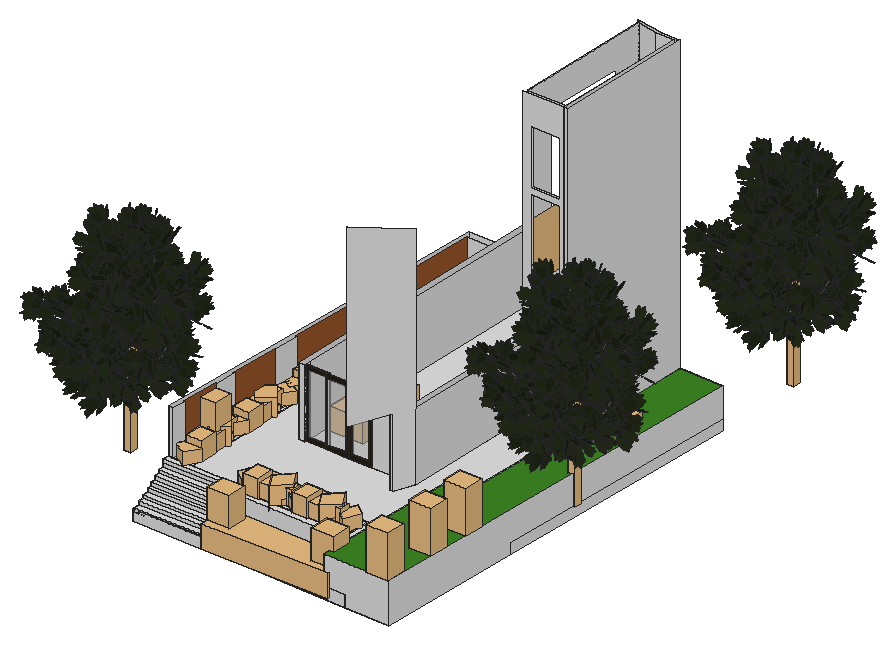
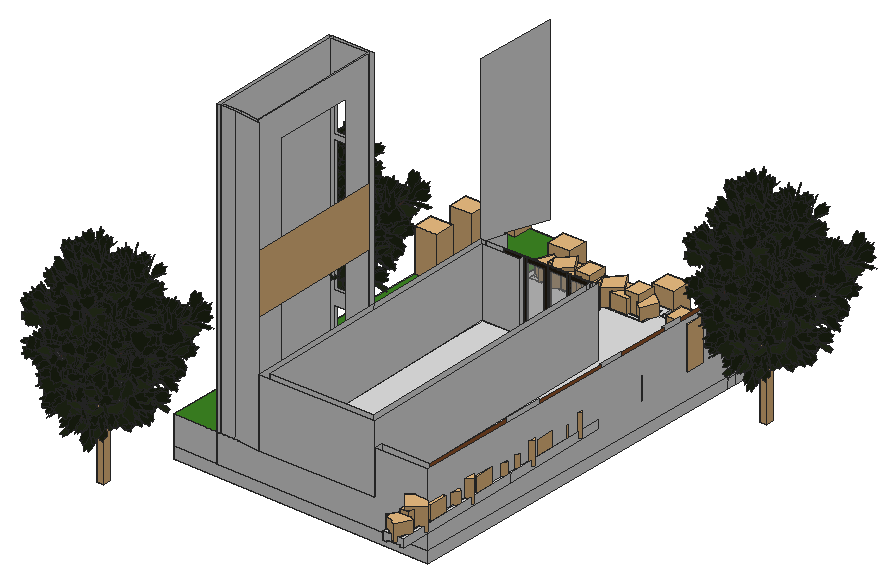
# SketchUp Ruby script. Lengths in inches.
U = 1.inch
M = Sketchup.active_model
def pt(a) = Geom::Point3d.new(a.map { |v| v * U })
def face(e, loops, mat)
  f = e.add_face(loops[0].map { |a| pt(a) })
  loops[1..].each { |l| e.add_face(l.map { |a| pt(a) }).erase! }
  f.material = f.back_material = mat if mat
  f
end
# faces: each face lists its corners as indices into pts; further lists are holes
def faces(e, pts, list, mat = nil) = list.each { |f| face(e, (f[0].is_a?(Array) ? f : [f]).map { |l| l.map { |i| pts[i] } }, mat) }
# xy, xz, yz: faces in a plane at the given z, y or x. An outline is a flat list of corners, or four numbers for a rectangle; further outlines are holes
def ring(l) = l.size == 4 ? [[l[0], l[1]], [l[2], l[1]], [l[2], l[3]], [l[0], l[3]]] : l.each_slice(2).to_a
def flat(e, list, mat, &to3) = list.each { |f| face(e, (f[0].is_a?(Array) ? f : [f]).map { |l| ring(l).map { |u, v| to3.(u, v) } }, mat) }
def xy(e, z, list, mat = nil) = flat(e, list, mat) { |x, y| [x, y, z] }
def xz(e, y, list, mat = nil) = flat(e, list, mat) { |x, z| [x, y, z] }
def yz(e, x, list, mat = nil) = flat(e, list, mat) { |y, z| [x, y, z] }
def lines(e, pts, list) = list.each { |a, b| e.add_line(pt(pts[a]), pt(pts[b])) }
# prism: a flat outline (further loops are holes) pulled along v
def prism(e, loops, v, mat = nil)
  f = face(e, loops, mat); d = Geom::Vector3d.new(v.map { |x| x * U })
  f.pushpull(f.normal.samedirection?(d) ? d.length : -d.length)
end
def box(e, o, s, mat = nil) = prism(e, [[o, [o[0] + s[0], o[1], o[2]], [o[0] + s[0], o[1] + s[1], o[2]], [o[0], o[1] + s[1], o[2]]]], [0, 0, s[2]], mat)
def at(x, y, z, deg = 0) = Geom::Transformation.translation(pt([x, y, z])) * Geom::Transformation.rotation(ORIGIN, Z_AXIS, deg.degrees)
def axes(o, x, y, z) = Geom::Transformation.new([*x, 0, *y, 0, *z, 0, *pt(o).to_a, 1])
def part(name) = M.definitions.add(name)
# library, detail: a bought-in or finely detailed component or shape, given as its bounding box
def library(name, o, s) = part(name).tap { |d| box(d.entities, o, s) }
def detail(e, o, s) = box(e.add_group.entities, o, s)
def put(e, d, t, mat = nil) = e.add_instance(d, t).tap { |i| i.material = mat if mat }
def group(e, t, mat = nil) = e.add_group.tap { |g| g.transformation = t; g.material = mat if mat }.entities
root = M.entities
M.materials.add("Green ash – green texture").color = [33, 41, 22]
M.materials.add("Material__1").color = [95, 70, 46]
M.materials.add("[Color A01]").color = [60, 133, 34]
M.materials.add("[Color M03]").color = [226, 226, 226]
M.materials.add("[Color_005]").color = [114, 114, 114]
M.materials.add("[Color_D09]").color = [86, 59, 49]
M.materials.add("[Translucent Glass Gray]2").color = [201, 201, 201]
M.materials["[Translucent Glass Gray]2"].alpha = 0.5
M.materials.add("[Wood Cherry Original]2").color = [152, 86, 42]
M.materials.add("oak swatch").color = [40, 31, 19]
c1 = part("Component\#13")
xz(c1.entities,0,[[2.54,0,9.87,0.64,10.99,2.07,11.4,3.42,15.13,2.28,14.48,4.31,16.14,5.21,16.14,6.08,19.81,7.28,19.6,9.67,17.45,11.49,17.45,12.16,18.82,14.37,17.48,14.37,14.41,13.66,14.41,15.23,12.5625,17.49,9.84,15.21,8.9,13.85,7.74,13.625,7.35,12.68,6.87,13.02,6.35,12.27,5.92,10.47,4.2,7.42,2.84,6.89,0,2.38,0.07,1.59,2.8125,4.94,3.37,3.59,2.54,3.37,2.12,2.22]],"Green ash – green texture")
c2 = part("Component\#14")
xz(c2.entities,0,[[1.1,0,1.61,0,2.73,1.11,4.34,2.72,5.21,6.36,5.85,7.16,6.35,6.9375,6.85,8.05,8.03,8.05,8.625,9.25,10.11,11.7,9.56,13.83,9.56,15.84,7.83,15.84,6.03,14.37,5.31,16.54,4.4375,17.39,1.45,14.31,0,9.15,1.4,5.18,3.01,6.08,1.98,1.39]],"Green ash – green texture")
c3 = part("Component\#16")
put(c3.entities,c1,axes([0,7.77,0],[1,0,0],[0,0.89571,0.44464],[0,-0.44464,0.89571]))
put(c3.entities,c2,axes([2.15,6.37,5.26],[0.57629,-0.80824,0.12095],[0.79263,0.51673,-0.3236],[0.19905,0.28236,0.93843]))
c4 = part("Component\#3")
put(c4.entities,c3,axes([-4.97,-3.22,4.05],[0.69883,-0.69034,0.18725],[0.53248,0.3273,-0.7806],[0.47759,0.64522,0.59632]))
c5 = part("Component\#4")
put(c5.entities,c4,axes([0,5.2,2.2],[1,0,0],[0,0.90259,0.43051],[0,-0.43051,0.90259]))
c6 = part("leaf group 2")
put(c6.entities,c5,axes([-11.99,4.41,-4.35],[2.22014,-0.82385,1.14017],[1.36501,1.77637,-1.37441],[-0.33979,1.75315,1.92841]))
c7 = part("Component\#5")
put(c7.entities,c6,axes([-5.27,11.65,1.68],[-0.48323,0.10636,-0.43072],[-0.11515,-0.64511,-0.03012],[-0.42845,0.05342,0.49388]))
c8 = part("Component\#15")
xz(c8.entities,0,[[0.64,0,0,0.1875,4.21,2.81,8.59,4.11,12.8,4.11,19.57,2.81,12.8,3.73,8.59,3.73,4.21,2.3125]],"[Color_D09]")
c9 = part("Leafy twig")
put(c9.entities,c7,axes([23.53,12.57,24.85],[0.06536,-0.90475,-0.42089],[0.61791,-0.2945,0.72901],[-0.78353,-0.30772,0.53981]))
put(c9.entities,c7,axes([22.7,12.25,24.83],[-0.47146,-0.89493,0.11311],[0.80135,-0.48549,-0.35888],[0.36776,-0.0521,0.90651]))
put(c9.entities,c7,axes([24.25,0.65,20.83],[0.8253,-0.50372,0.24924],[0.23848,0.71461,0.65749],[-0.51157,-0.48438,0.71194]))
put(c9.entities,c7,axes([23.54,-2.45,18.63],[0.04689,-0.92492,0.3511],[0.72122,-0.28285,-0.64421],[0.71641,0.2674,0.65188]))
put(c9.entities,c7,axes([22.39,16.15,27.04],[-0.5311,-0.82173,0.2419],[0.41574,0.01583,0.89559],[-0.77461,0.50499,0.40813]))
put(c9.entities,c8,axes([22.76,-5.09,13.48],[0,1.66539,0.44624],[-1.72414,0,0],[0,-0.44624,1.66539]))
c10 = part("Component\#12")
p = [[0,0,0.13],[0.41,0.77,0],[4.07,2.79,10.125],[3.73,2.15,10.23],[7.66,4.77,23.875],[7.4,4.27,23.96],
  [8.6875,5.26,35.99],[8.5,4.91,36.05],[8.32,4.9375,46.95],[8.21,4.74,46.98]]
faces(c10.entities,p,[[0,1,2,3],[3,2,4,5],[4,6,7,5],[6,8,9,7]],"[Color_005]")
c11 = part("Component\#2")
put(c11.entities,c10,axes([3.13,0.17,-0.45],[3.38032,6.88592,0.52481],[-5.85488,3.97559,0.303],[0,-1.35912,3.54524]))
put(c11.entities,c7,axes([0.37,31.375,148.94],[0.47772,0.64064,-1.51139],[2.85768,-0.62659,0.20284],[-0.43926,-3.3797,-0.3241]))
c12 = part("Tree branch")
put(c12.entities,c9,axes([28.11,72.66,46.26],[0.77413,-0.41274,-0.47998],[0.6311,0.56229,0.53435],[0.04934,-0.71657,0.69577]))
put(c12.entities,c9,axes([31.25,3.94,9.17],[0.73236,0.67893,0.05208],[-0.46223,0.55185,-0.69413],[-0.5,0.48428,0.71797]))
put(c12.entities,c9,axes([20.16,84.84,57.95],[0.96628,0.19619,0.16678],[-0.2575,0.73909,0.62245],[-0.00115,-0.6444,0.76469]))
put(c12.entities,c9,axes([30.13,29.18,11.93],[0.86603,0.2796,0.41452],[0,0.82904,-0.55919],[-0.5,0.48428,0.71797]))
put(c12.entities,c9,axes([47.67,28.63,-3.7],[0.1205,-0.71255,0.69119],[0.96646,0.24327,0.08231],[-0.2268,0.65809,0.71797]))
put(c12.entities,c9,axes([48.76,50.64,76.31],[-0.6716,0.46861,-0.57389],[0.01402,0.78248,0.62252],[0.74078,0.41004,-0.53209]))
put(c12.entities,c11,axes([42.34,0,10.34],[0.39368,0,0],[0,0.22544,-0.24092],[0,0.54032,0.50562]))
put(c12.entities,c9,axes([64.51,80.82,101.08],[-0.99604,0.06562,-0.06004],[-0.0106,0.58266,0.81265],[0.08831,0.81006,-0.57966]))
c13 = library("Component\#7",[-6.35,9.4375,-76.57],[12.56,13.68,315.77])
c14 = part("Component\#9")
put(c14.entities,c9,axes([-3.64,36.17,23.18],[0.95801,0.10249,0.26779],[-0.28581,0.41631,0.86313],[-0.02302,-0.90343,0.42812]))
put(c14.entities,c9,axes([13.16,55.79,39.92],[0.70711,-0.61725,0.34497],[0,0.48786,0.87292],[-0.70711,-0.61725,0.34497]))
put(c14.entities,c11,axes([18.8125,5.17,0.46],[0.25503,0,0],[0,0.20007,-0.0752],[0,0.16866,0.44872]))
put(c14.entities,c9,axes([23.62,-10.17,21.5],[-0.56253,0.81775,0.12181],[0.38738,0.13053,0.91263],[0.73041,0.56057,-0.39021]))
put(c14.entities,c9,axes([45.18,27.18,68.96],[-0.96593,-0.22593,0.12627],[0.12295,0.02876,0.992],[-0.22775,0.97372,0]))
c15 = part("Component\#10")
put(c15.entities,c11,axes([21.47,3.93,0.22],[0.25503,0,0],[0,0.21068,-0.03601],[0,0.08077,0.47252]))
put(c15.entities,c9,axes([-4.05,13.6875,55.34],[0.70711,0.70373,-0.069],[0,0.09758,0.99523],[0.70711,-0.70373,0.069]))
put(c15.entities,c9,axes([6.52,33.54,18.07],[0.92587,-0.37604,0.03687],[0,0.09758,0.99523],[-0.37784,-0.92145,0.09035]))
c16 = part("Component\#11")
put(c16.entities,c9,axes([26.17,74.02,40.56],[0.25882,-0.64004,0.72344],[0,0.74896,0.66262],[-0.96593,-0.1715,0.19384]))
put(c16.entities,c9,axes([6.38,24.03,55.81],[-0.04786,0.8645,-0.50035],[0.15558,0.50126,0.85119],[0.98666,-0.03711,-0.15849]))
put(c16.entities,c11,axes([17.68,0,1.01],[0.32282,0,0],[0,0.21407,-0.16545],[0,0.37107,0.48011]))
put(c16.entities,c9,axes([-9.1875,31.15,28.07],[0.82314,0.37626,-0.42529],[0,0.74896,0.66262],[0.56784,-0.54543,0.61649]))
put(c16.entities,c9,axes([0.54,-12.07,9.94],[0.19622,0.90478,-0.37799],[-0.67396,0.40444,0.61823],[0.71224,0.13344,0.68914]))
put(c16.entities,c9,axes([7.34,9.15,39.57],[0.05153,0.73872,-0.67204],[0.38679,0.60565,0.6954],[0.92072,-0.29578,-0.25452]))
put(c16.entities,c9,axes([36.2,51.23,15.73],[-0.18626,-0.35374,0.91661],[-0.31641,0.90483,0.2849],[-0.93016,-0.23696,-0.28046]))
c17 = part("Tree")
put(c17.entities,c12,axes([-22.29,52.36,216.76],[0.38964,-1.07313,-0.10036],[1.06809,0.37236,0.19631],[-0.13881,-0.14712,1.22884]))
put(c17.entities,c12,axes([59.83,6.78,230.57],[-1.28826,-0.23008,-0.3647],[0.05148,-1.22938,0.51215],[-0.34663,0.55136,1.25774]))
put(c17.entities,c13,axes([-2.16,-18.04,104.22],[1.30157,0,0],[0,1.30157,0],[0,0,1.36111]))
put(c17.entities,c12,axes([-55.8,4.2,115.32],[1.30157,0,0],[0,1.29536,0.19359],[0,-0.26855,1.38538]))
put(c17.entities,c12,axes([5.36,-52.22,156.04],[-0.23532,1.19719,-0.71362],[-1.32974,0,0.39335],[0.40758,0.6912,1.23603]))
put(c17.entities,c14,axes([-20.09,22.57,317.7],[0,-1.33697,0],[1.33697,0,0],[0,0,1.4573]))
put(c17.entities,c12,axes([44.2,-31.84,172.82],[-1.11894,0.85085,0],[-0.85085,-1.11894,0],[0,0,1.53221]))
put(c17.entities,c12,axes([-10.2,63.7,119.93],[0.28716,-1.46366,0],[1.41378,0.27737,0.38604],[-0.41292,-0.08101,1.5704]))
put(c17.entities,c12,axes([-29.03,-40.72,232.79],[0.5211,0.98898,-0.38718],[-1.02974,0.58664,0.11255],[0.35577,0.28216,1.19957]))
put(c17.entities,c12,axes([44.92,21.7,135.38],[-1.05627,-0.44294,0],[0.44294,-1.05627,0],[0,0,1.24847]))
put(c17.entities,c14,axes([-32.94,-0.59,304.82],[1.2814,-0.22825,0],[0.22825,1.2814,0],[0,0,1.41871]))
put(c17.entities,c14,axes([0.6,-31.29,315.98],[0.13082,1.33422,0],[-1.33422,0.13082,0],[0,0,1.46127]))
put(c17.entities,c14,axes([21.3,1.66,315.16],[-1.25722,0.32198,-0.09905],[-0.32539,-1.26867,0.00612],[-0.08719,0.09194,1.40547]))
put(c17.entities,c15,axes([-19,30.84,372.72],[0.65078,-1.12719,0],[1.12719,0.65078,0],[0,0,1.41871]))
put(c17.entities,c15,axes([14.39,-16.125,357],[-0.73695,1.06095,0.15933],[-1.03698,-0.75397,0.2242],[0.29981,0,1.38667]))
put(c17.entities,c16,axes([-5.9,-20.03,270.39],[0,1.47598,0],[-1.4157,0,0.41751],[0.45509,0,1.54311]))
put(c17.entities,c16,axes([-18.4375,22.18,263.88],[0.84243,-1.42226,-0.32685],[1.40385,0.7063,0.64743],[-0.37678,-0.54841,1.68147]))
put(c17.entities,c16,axes([-29.32,4.9,283.41],[1.35363,0,0],[0,1.33841,0.20242],[0,-0.22063,1.45887]))
put(c17.entities,c16,axes([17.31,11.65,257.52],[-1.14969,-0.5642,-0.25322],[0.46017,-1.12719,0.50159],[-0.40066,0.32434,1.3027]))
put(c17.entities,c16,axes([16.3,15.3125,240.45],[-0.98541,-0.85203,0.68095],[1.00747,-1.01506,0.22317],[0.31818,0.5753,1.40228]))
put(c17.entities,c12,axes([-46.75,22.93,206.12],[1.08363,-0.37101,0],[0.37101,1.08363,0],[0,0,1.24847]))
put(c17.entities,c12,axes([41.1,-35.18,99.125],[-1.05556,0.85173,0.25344],[-0.84493,-1.04965,0.12953],[0.39153,-0.09409,1.38106]))
c18 = library("Group\#13",[19.84,-0.11,0],[59.32,169.94,39.58])
c19 = library("Yukka",[-2.74,-1.93,0],[38.67,34.64,74.8125])
c20 = library("Areca palm plant",[0,0,0],[49.1,36.6,54.46])
c21 = library("Group\#74",[-84.69,-90.07,-0.36],[176.51,175.13,171.4])
c22 = library("Group\#130",[-7.34,-1.2,0],[38.67,35.81,49.04])
c23 = library("Group20\#1",[-20.81,-17.08,3.79],[39.86,39.43,37.51])
c24 = library("Group38\#2",[14.01,28.44,-23.43],[18.58,18.32,38.89])
c25 = part("Group\#8")
xy(c25.entities,0,[[0,0,6,234.8],[30,0,36,234.8]])
xy(c25.entities,3,[[6,0,30,234.8]])
xy(c25.entities,7,[[6,5,30,229.8]],"Material__1")
xy(c25.entities,15,[[[0,0,36,234.8],[6,5,30,229.8]]])
xz(c25.entities,0,[[0,0,6,0,6,3,30,3,30,0,36,0,36,15,0,15]])
xz(c25.entities,5,[[6,7,30,15]])
xz(c25.entities,229.8,[[6,7,30,15]])
xz(c25.entities,234.8,[[0,0,0,15,36,15,36,0,30,0,30,3,6,3,6,0]])
yz(c25.entities,0,[[0,0,234.8,15]])
yz(c25.entities,6,[[0,0,234.8,3],[5,7,229.8,15]])
yz(c25.entities,30,[[0,0,234.8,3],[5,7,229.8,15]])
yz(c25.entities,36,[[0,0,234.8,15]])
c26 = part("Group\#9")
put(c26.entities,c20,axes([-6.2,56.6,6.08],[0.45017,-0.56191,0],[0.66137,0.52986,0],[0,0,0.72]))
put(c26.entities,c20,axes([-6.2,158.41,6.08],[0.45017,-0.56191,0],[0.66137,0.52986,0],[0,0,0.72]))
put(c26.entities,c21,axes([14.93,193.18,6.05],[-0.04961,-0.08593,0],[0.08593,-0.04961,0],[0,0,0.10522]))
put(c26.entities,c21,axes([14.93,44.05,6.05],[-0.04961,-0.08593,0],[0.08593,-0.04961,0],[0,0,0.10522]))
put(c26.entities,c21,axes([14.93,71.3,6.05],[-0.04961,-0.08593,0],[0.08593,-0.04961,0],[0,0,0.10522]))
put(c26.entities,c22,axes([24.9375,89.91,8],[0,0.79,0],[-0.79,0,0],[0,0,0.79]))
put(c26.entities,c21,axes([14.93,91.37,6.05],[-0.04961,-0.08593,0],[0.08593,-0.04961,0],[0,0,0.10522]))
put(c26.entities,c21,axes([17.19,15.79,6.07],[-0.08133,-0.14087,0],[0.14087,-0.08133,0],[0,0,0.1725]))
put(c26.entities,c21,axes([17.19,121.23,6.07],[-0.08133,-0.14087,0],[0.14087,-0.08133,0],[0,0,0.1725]))
put(c26.entities,c21,axes([17.19,223.04,6.07],[-0.08133,-0.14087,0],[0.14087,-0.08133,0],[0,0,0.1725]))
put(c26.entities,c21,axes([14.93,145.87,6.05],[-0.04961,-0.08593,0],[0.08593,-0.04961,0],[0,0,0.10522]))
put(c26.entities,c23,axes([18.97,181.79,4.77],[0,0.85,0],[-0.85,0,0],[0,0,0.85]))
put(c26.entities,c24,axes([-4.1,100.66,28.17],[0.8848,0,0],[0,0.94674,0],[0,0,0.85826]))
put(c26.entities,c25,at(0,0,0))
put(c26.entities,c22,axes([24.9375,191.72,8],[0,0.79,0],[-0.79,0,0],[0,0,0.79]))
put(c26.entities,c24,axes([-4.1,-1.15,28.17],[0.8848,0,0],[0,0.94674,0],[0,0,0.85826]))
put(c26.entities,c21,axes([14.93,173.12,6.05],[-0.04961,-0.08593,0],[0.08593,-0.04961,0],[0,0,0.10522]))
put(c26.entities,c23,axes([18.97,79.98,4.77],[0,0.85,0],[-0.85,0,0],[0,0,0.85]))
c27 = part("Group\#10")
put(c27.entities,c20,axes([-6.2,56.6,6.08],[0.45017,-0.56191,0],[0.66137,0.52986,0],[0,0,0.72]))
put(c27.entities,c20,axes([-6.2,158.41,6.08],[0.45017,-0.56191,0],[0.66137,0.52986,0],[0,0,0.72]))
put(c27.entities,c21,axes([14.93,193.18,6.05],[-0.04961,-0.08593,0],[0.08593,-0.04961,0],[0,0,0.10522]))
put(c27.entities,c21,axes([14.93,44.05,6.05],[-0.04961,-0.08593,0],[0.08593,-0.04961,0],[0,0,0.10522]))
put(c27.entities,c21,axes([14.93,71.3,6.05],[-0.04961,-0.08593,0],[0.08593,-0.04961,0],[0,0,0.10522]))
put(c27.entities,c22,axes([24.9375,89.91,8],[0,0.79,0],[-0.79,0,0],[0,0,0.79]))
put(c27.entities,c21,axes([14.93,91.37,6.05],[-0.04961,-0.08593,0],[0.08593,-0.04961,0],[0,0,0.10522]))
put(c27.entities,c21,axes([17.19,15.79,6.07],[-0.08133,-0.14087,0],[0.14087,-0.08133,0],[0,0,0.1725]))
put(c27.entities,c21,axes([17.19,121.23,6.07],[-0.08133,-0.14087,0],[0.14087,-0.08133,0],[0,0,0.1725]))
put(c27.entities,c21,axes([17.19,223.04,6.07],[-0.08133,-0.14087,0],[0.14087,-0.08133,0],[0,0,0.1725]))
put(c27.entities,c21,axes([14.93,145.87,6.05],[-0.04961,-0.08593,0],[0.08593,-0.04961,0],[0,0,0.10522]))
put(c27.entities,c23,axes([18.97,181.79,4.77],[0,0.85,0],[-0.85,0,0],[0,0,0.85]))
put(c27.entities,c24,axes([-4.1,100.66,28.17],[0.8848,0,0],[0,0.94674,0],[0,0,0.85826]))
put(c27.entities,c25,at(0,0,0))
put(c27.entities,c22,axes([24.9375,191.72,8],[0,0.79,0],[-0.79,0,0],[0,0,0.79]))
put(c27.entities,c24,axes([-4.1,-1.15,28.17],[0.8848,0,0],[0,0.94674,0],[0,0,0.85826]))
put(c27.entities,c21,axes([14.93,173.12,6.05],[-0.04961,-0.08593,0],[0.08593,-0.04961,0],[0,0,0.10522]))
put(c27.entities,c23,axes([18.97,79.98,4.77],[0,0.85,0],[-0.85,0,0],[0,0,0.85]))
c28 = library("Dome Light",[-12,-12,0],[24,24,12])
c29 = part("Group\#6")
box(c29.entities,[0,0,0],[1.77,4.72,80.31],"oak swatch")
c30 = part("Exterior Sliding Doors")
xy(c30.entities,0,[[1.77,33.07,3.54,70.87],[1.77,70.87,3.54,108.66]])
xy(c30.entities,0,[[0,0,1.77,33.07],[0,108.66,1.77,141.73]],"oak swatch")
xy(c30.entities,4.72,[[0,4.72,1.77,33.07],[1.77,37.8,3.54,66.14],[1.77,75.88,3.54,103.9375],[0,108.66,1.77,137.01]],"oak swatch")
xy(c30.entities,75.59,[[1.77,37.8,3.54,66.14],[1.77,75.88,3.54,103.9375]])
xy(c30.entities,75.59,[[0,4.72,1.77,33.07],[0,108.66,1.77,137.01]],"oak swatch")
xy(c30.entities,80.31,[[0,0,1.77,33.07],[1.77,33.07,3.54,70.87],[1.77,70.87,3.54,108.66],[0,108.66,1.77,141.73]],"oak swatch")
xz(c30.entities,0,[[0,0,1.77,80.31]],"oak swatch")
xz(c30.entities,4.72,[[0,4.72,1.77,75.59]],"oak swatch")
xz(c30.entities,33.07,[[0,0,1.77,4.72],[1.77,0,3.54,80.31],[0,75.59,1.77,80.31]],"oak swatch")
xz(c30.entities,37.8,[[1.77,4.72,3.54,75.59]])
xz(c30.entities,66.14,[[1.77,4.72,3.54,75.59]],"oak swatch")
xz(c30.entities,70.87,[[1.77,0,3.54,80.31]])
xz(c30.entities,75.88,[[1.77,4.72,3.54,75.59]])
xz(c30.entities,103.9375,[[1.77,4.72,3.54,75.59]],"oak swatch")
xz(c30.entities,108.66,[[1.77,4.72,3.54,75.59]])
xz(c30.entities,108.66,[[0,0,3.54,4.72],[0,75.59,3.54,80.31]],"oak swatch")
xz(c30.entities,137.01,[[0,4.72,1.77,75.59]],"oak swatch")
xz(c30.entities,141.73,[[0,0,1.77,80.31]],"oak swatch")
yz(c30.entities,0,[[0,0,33.07,0,33.07,4.72,4.72,4.72,4.72,75.59,33.07,75.59,33.07,80.31,0,80.31],[108.66,0,141.73,0,141.73,80.31,108.66,80.31,108.66,75.59,137.01,75.59,137.01,4.72,108.66,4.72]],"oak swatch")
yz(c30.entities,1.77,[[4.72,4.72,33.07,75.59],[37.8,4.72,66.14,75.59],[75.88,4.72,103.9375,75.59],[108.66,4.72,137.01,75.59]],"[Translucent Glass Gray]2")
yz(c30.entities,1.77,[[0,0,33.07,0,33.07,4.72,4.72,4.72,4.72,75.59,33.07,75.59,33.07,80.31,0,80.31],[[33.07,0,70.87,80.31],[37.8,4.72,66.14,75.59]],[[70.87,0,141.73,80.31],[108.66,4.72,137.01,75.59],[75.88,4.72,103.9375,75.59]]],"oak swatch")
yz(c30.entities,3.54,[[[33.07,0,70.87,80.31],[37.8,4.72,66.14,75.59]],[[70.87,0,108.66,80.31],[75.88,4.72,103.9375,75.59]]],"oak swatch")
put(c30.entities,c29,at(0,33.07,0))
put(c30.entities,c29,at(0,103.9375,0))
c31 = library("Sofá",[11.66,3.97,0],[59.11,123.04,38.06])
c32 = library("Mesh Light\#10",[-0.5,-0.5,-0.1],[1,1,0.2])
xy(root,-25.27,[[688.83,0,610.92,2.02,612.22,52.03,617.61,259.48,695.52,257.46],[610.92,2.02,354.33,8.68,355.63,58.69,573.07,53.05,612.22,52.03],[354.25,5.69,233.32,8.83,234.92,70.58,355.86,67.4375,355.63,58.69,354.33,8.68],[612.22,52.03,573.07,53.05,578.46,260.5,617.61,259.48],[573.07,53.05,355.63,58.69,355.86,67.4375,356.2,80.62,235.26,83.76,251.84,722.48,707.28,710.66,695.52,257.46,617.61,259.48,578.46,260.5],
  [355.86,67.4375,234.92,70.58,235.26,83.76,356.2,80.62]],"[Color M03]")
xy(root,-9.18,[[235.26,8.63,235.26,84.72,356.2,84.72,356.2,80.62,355.86,67.4375,355.63,58.69,354.33,8.68,354.33,8.63],[354.33,8.63,354.33,8.68,355.63,58.69,355.86,67.4375,356.2,80.62,356.2,8.63]],"[Color M03]")
xy(root,-5.71,[[610.92,2.02,612.22,52.03,573.07,53.05,571.77,3.04],[571.77,3.04,573.07,53.05,355.63,58.69,354.33,8.68,356.2,8.63],[354.25,5.69,354.33,8.68,355.63,58.69,355.86,67.4375,234.92,70.58,233.32,8.83],[612.22,52.03,617.61,259.48,578.46,260.5,573.07,53.05],[573.07,53.05,578.46,260.5,617.61,259.48,629.37,712.68,251.84,722.48,235.26,83.76,356.2,80.62,355.86,67.4375,355.63,58.69],
  [355.86,67.4375,356.2,80.62,235.26,83.76,234.92,70.58],[695.52,257.46,617.61,259.48,629.37,712.68,707.28,710.66]],"[Color M03]")
xy(root,-3.18,[[235.26,8.63,356.2,19.63]],"[Color M03]")
xy(root,2.82,[[235.26,19.63,356.2,28.2]],"[Color M03]")
xy(root,8.82,[[235.26,28.2,356.2,38.38]],"[Color M03]")
xy(root,14.82,[[235.26,38.38,356.2,44.38]],"[Color M03]")
xy(root,20.82,[[235.26,44.38,356.2,53.07]],"[Color M03]")
xy(root,23.73,[[365.76,68.16,564.82,109.59]],"[Color M03]")
xy(root,27.42,[[235.26,53.07,356.2,61.88]],"[Color M03]")
xy(root,33.42,[[235.26,61.88,356.2,71.76]],"[Color M03]")
xy(root,45.29,[[688.83,0,707.28,710.66,629.37,712.68,617.61,259.48,578.46,260.5,573.07,53.05,571.77,3.04]],"[Color A01]")
xy(root,45.42,[[[573.07,53.05,578.46,260.5,617.61,259.48,622.99,466.93,550.5,466.93,550.5,232.04,537.14,200.35,536.83,199.61,530.83,199.61,537.63,219.1875,537.97,232.04,473.11,232.04,473.11,242.84,356.8,242.84,356.8,232.04,346,232.04,346,720.04,345.63,706.05,278.13,707.8,260.27,708.27,256.05,546.04,256.62,546.02,254.77,475.04,254.21,475.06,250.87,346.18,251.43,346.17,250.22,299.74,249.66,299.75,247.39,212.16,248.39,212.13,247.41,174.67,246.41,174.7,244.68,107.8,244.05,83.53,356.2,80.62,356.2,71.76,355.97,71.76,355.63,58.69],[365.76,68.16,564.82,109.59]],[235.26,71.76,355.97,71.76,356.2,80.62,244.05,83.53,235.26,83.76],[355.97,71.76,356.2,71.76,356.2,80.62],[244.68,107.8,246.41,174.7,245.35,174.72,243.62,107.83],[247.41,174.67,248.39,212.13,247.39,212.16,246.41,174.7],
  [530.83,199.61,537.63,219.1875,537.14,200.35,536.83,199.61],[537.14,200.35,550.5,232.04,542.1,232.04,537.63,219.1875],[247.39,212.16,249.66,299.75,248.6,299.78,246.32,212.18],[537.63,219.1875,542.1,232.04,537.97,232.04],[346,232.04,356.8,232.04,356.8,709.23,539.69,709.23,539.69,298.57,550.5,714.73,346,720.04],
  [473.11,232.04,537.97,232.04,538.25,242.84,473.11,242.84],[537.97,232.04,550.5,232.04,550.5,714.73,539.69,298.57,539.69,242.84,538.25,242.84],[356.8,242.84,538.25,242.84,539.69,298.57,539.69,709.23,356.8,709.23],[538.25,242.84,539.69,242.84,539.69,298.57],[250.22,299.74,251.43,346.17,250.87,346.18,249.66,299.75],
  [250.87,346.18,254.21,475.06,253.15,475.08,249.8,346.21],[550.5,466.93,584.24,466.93,584.375,472.23,555.8,472.23,555.8,713.83,590.5,708.34,590.64,713.6875,550.5,714.73],[584.24,466.93,584.375,472.23,622.99,472.23,622.99,466.93],[622.99,466.93,622.99,472.23,623.13,472.23,623.13,708.16,622.99,708.16,622.99,712.68,629.37,712.68,623.13,472.23],[622.99,466.93,622.99,712.68,629.37,712.68,623.13,472.23],
  [622.99,466.93,623.13,472.23,629.37,712.68,629.37,466.93],[555.8,472.23,584.375,472.23,590.5,708.34,555.8,713.83],[584.375,472.23,622.99,472.23,622.99,708.16,591.7,708.16,590.5,708.34],[622.99,472.23,623.13,708.16],[254.77,475.04,256.62,546.02,256.05,546.04,254.21,475.06],
  [256.05,546.04,260.27,708.27,259.2,708.3,254.99,546.0625],[278.13,707.8,278.14,708.3,260.28,708.76,260.27,708.27],[591.7,708.16,590.5,708.34,590.64,713.6875,597,712.68,622.99,712.68,622.99,708.16],[597,712.68,629.37,712.68,590.64,713.6875],[590.64,713.6875,550.5,714.73,550.5,720.04],
  [550.5,714.73,346,720.04,550.5,720.04]],"[Color M03]")
xz(root,8.63,[[235.26,-9.18,356.2,-3.18]],"[Color M03]")
xz(root,19.63,[[235.26,-3.18,356.2,2.82]],"[Color M03]")
xz(root,28.2,[[235.26,2.82,356.2,8.82]],"[Color M03]")
xz(root,38.38,[[235.26,8.82,356.2,14.82]],"[Color M03]")
xz(root,44.38,[[235.26,14.82,356.2,20.82]],"[Color M03]")
xz(root,53.07,[[235.26,20.82,356.2,27.42]],"[Color M03]")
xz(root,61.88,[[235.26,27.42,356.2,33.42]],"[Color M03]")
xz(root,68.16,[[365.76,23.73,564.82,45.42]],"[Color M03]")
xz(root,71.76,[[235.26,33.42,356.2,39.42],[235.26,39.42,356.2,45.42]],"[Color M03]")
xz(root,109.59,[[365.76,23.73,564.82,45.42]],"[Color M03]")
xz(root,199.61,[[530.83,45.42,536.83,165.42]],"[Color M03]")
xz(root,232.04,[[346,45.42,356.8,165.42],[473.11,45.42,542.1,165.42],[542.1,45.42,550.5,165.42]],"[Color M03]")
xz(root,242.84,[[473.11,45.42,539.69,165.42]],"[Color M03]")
xz(root,466.93,[[[550.5,45.42,622.99,561.04],[564.58,167.67,616.16,404.08],[564.45,412.95,616.16,510.7],[563.22,53.02,616.16,144.21]],[622.99,45.42,629.37,561.04]],"[Color M03]")
xz(root,472.23,[[[555.8,45.42,623.13,561.04],[564.58,167.67,616.16,404.08],[564.45,412.95,616.16,510.7],[563.22,53.02,616.16,144.21]]],"[Color M03]")
xz(root,708.16,[[591.7,45.42,623.13,561.04]],"[Color M03]")
xz(root,709.23,[[356.8,45.42,539.69,165.42]],"[Color M03]")
xz(root,712.68,[[597,45.42,622.99,561.04],[622.99,45.42,629.37,561.04]],"[Color M03]")
xz(root,720.04,[[346,45.42,550.5,165.42]],"[Color M03]")
yz(root,235.26,[[8.63,-9.18,8.63,-3.18,19.63,-3.18,19.63,2.82,28.2,2.82,28.2,8.82,38.38,8.82,38.38,14.82,44.38,14.82,44.38,20.82,53.07,20.82,53.07,27.42,61.88,27.42,61.88,33.42,71.76,33.42,71.76,45.42,83.76,45.42,83.76,-9.18],[83.76,-9.18,83.76,-5.71,84.72,-9.18]],"[Color M03]")
yz(root,346,[[232.04,45.42,720.04,165.42]],"[Color M03]")
yz(root,356.2,[[8.63,-9.18,80.62,-9.18,80.62,45.42,71.76,45.42,71.76,33.42,61.88,33.42,61.88,27.42,53.07,27.42,53.07,20.82,44.38,20.82,44.38,14.82,38.38,14.82,38.38,8.82,28.2,8.82,28.2,2.82,19.63,2.82,19.63,-3.18,8.63,-3.18]],"[Color M03]")
yz(root,356.8,[[232.04,45.42,242.84,45.42,232.49,165.42,232.04,165.42],[242.84,45.42,242.84,165.42,232.49,165.42],[242.84,45.42,709.23,165.42]],"[Color M03]")
yz(root,365.76,[[68.16,23.73,109.59,45.42]],"[Color M03]")
yz(root,473.11,[[232.04,45.42,242.84,165.42]],"[Color M03]")
yz(root,539.69,[[242.84,45.42,709.23,165.42]],"[Color M03]")
yz(root,550.5,[[232.04,45.42,466.93,165.42],[466.93,45.42,720.04,165.42]],"[Color M03]")
yz(root,555.8,[[[470.93,44.11,715.14,562.35],[472.23,45.42,713.83,561.04]]],"[Color M03]")
yz(root,564.82,[[68.16,23.73,109.59,45.42]],"[Color M03]")
yz(root,622.99,[[466.93,45.42,712.68,561.04]],"[Color M03]")
yz(root,623.13,[[472.23,45.42,708.16,561.04]],"[Color M03]")
yz(root,629.37,[[466.93,45.42,712.68,561.04]],"[Color M03]")
p = [[571.77,3.04,-5.71],[610.92,2.02,-5.71],[610.92,2.02,-25.27],[688.83,0,-25.27],[688.83,0,45.29],[571.77,3.04,45.29],
  [695.52,257.46,-5.71],[707.28,710.66,-5.71],[707.28,710.66,45.29],[695.52,257.46,-25.27],[356.2,8.63,-5.71],[354.33,8.68,-5.71],
  [354.33,8.68,-9.18],[354.33,8.68,-25.27],[612.22,52.03,-25.27],[612.22,52.03,-5.71],[354.25,5.69,-5.71],[233.32,8.83,-5.71],
  [233.32,8.83,-9.18],[233.32,8.83,-25.27],[354.25,5.69,-25.27],[354.25,5.69,-9.18],[354.33,8.63,-9.18],[355.63,58.69,-9.18],
  [355.63,58.69,-25.27],[234.92,70.58,-9.18],[234.92,70.58,-25.27],[573.07,53.05,-5.71],[573.07,53.05,-25.27],[617.61,259.48,-5.71],
  [617.61,259.48,-25.27],[355.63,58.69,-5.71],[578.46,260.5,-5.71],[578.46,260.5,-25.27],[355.86,67.4375,-25.27],[355.86,67.4375,-9.18],
  [234.92,70.58,-5.71],[355.86,67.4375,-5.71],[356.2,80.62,-9.18],[356.2,80.62,-25.27],[235.26,83.76,-9.18],[235.26,83.76,-25.27],
  [235.26,83.76,-5.71],[356.2,80.62,-5.71],[251.84,722.48,-5.71],[251.84,722.48,-25.27],[707.28,710.66,-25.27],[629.37,712.68,-5.71],
  [235.26,84.72,-9.18],[356.2,83.76,-5.71],[356.2,84.72,-9.18],[573.07,53.05,45.29],[573.07,53.05,45.42],[355.63,58.69,45.42],
  [578.46,260.5,45.29],[356.2,80.62,45.42],[355.97,71.76,45.42],[244.05,83.53,45.42],[235.26,83.76,45.42],[251.84,722.48,123.23],
  [235.26,83.76,123.23],[617.61,259.48,45.29],[629.37,712.68,45.29],[346,720.04,45.42],[550.5,714.73,45.42],[590.64,713.6875,45.42],
  [629.37,712.68,45.42],[346,720.04,123.23],[541.98,211.82,44.68],[550.5,232.04,45.42],[537.14,200.35,45.42],[536.83,199.61,45.42],
  [536.83,199.61,43.67],[578.46,260.5,45.42],[617.61,259.48,45.42],[623.13,472.23,45.42],[622.99,466.93,45.42],[244.05,83.53,123.23],
  [244.68,107.8,45.42],[244.68,107.8,123.23],[243.62,107.83,45.42],[245.35,174.72,45.42],[245.35,174.72,123.23],[243.62,107.83,123.23],
  [550.5,232.04,328.48],[550.5,232.04,447.16],[508.8,133.09,479.92],[508.8,133.09,165.42],[536.83,199.61,165.42],[550.5,232.04,165.42],
  [550.5,232.04,171.42],[550.5,232.04,306.98],[246.41,174.7,45.42],[247.41,174.67,45.42],[247.41,174.67,123.23],[248.39,212.13,45.42],
  [248.39,212.13,123.23],[530.83,199.61,165.42],[542.1,232.04,165.42],[542.1,232.04,45.42],[537.63,219.1875,45.42],[530.83,199.61,45.42],
  [246.32,212.18,45.42],[246.32,212.18,123.23],[247.39,212.16,45.42],[248.6,299.78,45.42],[248.6,299.78,123.23],[249.66,299.75,45.42],
  [250.22,299.74,45.42],[250.22,299.74,123.23],[251.43,346.17,45.42],[251.43,346.17,123.23],[249.8,346.21,45.42],[253.15,475.08,45.42],
  [253.15,475.08,123.23],[249.8,346.21,123.23],[250.87,346.18,45.42],[254.21,475.06,45.42],[254.77,475.04,45.42],[254.77,475.04,123.23],
  [256.62,546.02,45.42],[256.62,546.02,123.23],[254.99,546.0625,45.42],[254.99,546.0625,123.23],[256.05,546.04,45.42],[259.2,708.3,123.23],
  [259.2,708.3,45.42],[260.27,708.27,45.42],[278.13,707.8,45.42],[345.63,706.05,45.42],[345.63,706.05,123.23],[590.5,708.34,45.42],
  [591.7,708.16,45.42],[591.7,708.16,561.04],[555.8,713.83,561.04],[555.8,713.83,45.42],[597,712.68,45.42],[550.5,720.04,45.42],
  [550.5,720.04,165.42],[550.5,720.04,171.42],[550.5,720.04,306.98],[550.5,720.04,328.48],[550.5,720.04,561.04],[597,712.68,561.04],
  [356.2,83.76,45.42]]
faces(root,p,[[0,1,2,3,4,5],[6,7,8,4,3,9],[1,0,10,11,12,13,2],[14,15,1,2],[16,17,18,19,20,21],[20,13,12,22,21],[13,12,23,24],[25,26,19,18],
  [27,28,14,15],[29,15,14,30],[31,27,28,24,23],[27,32,33,28],[23,24,34,35],[36,37,35,34,26,25],[38,39,34,35],[40,41,26,25],
  [42,43,38,39,41,40],[42,44,45,41,40],[29,30,9,6],[7,6,9,46],[29,32,33,30],[44,47,7,46,45],[22,12,11,16,21],[31,23,12,11],
  [36,25,18,17],[35,37,31,23],[43,38,35,37],[42,40,25,36],[48,42,49,50],[5,51,27,0],[31,27,51,52,53],[32,54,51,27],
  [55,43,37,31,53,56],[42,43,55,57,58],[59,44,42,58,60],[29,61,54,32],[29,47,62,61],[7,47,62,8],[63,64,65,66,62,47,44,59,67],[68,69,70,71,72],
  [52,51,54,73],[73,54,61,74],[74,61,62,66,75,76],[58,57,77,60],[77,57,78,79],[80,83,79,78],[84,85,86,87,88,71,70,69,89,90,91],[82,81,92,93,94],
  [93,95,96,94],[97,98,99,100,101],[102,103,96,95,104],[106,105,107,108,109],[108,110,111,109],[112,115,111,110,116],[114,113,117,118,119],[118,120,121,119],
  [122,123,121,120,124],[125,126,127,128,129,130],[67,130,129,63],[131,132,133,134,135],[136,65,137,138,139,140,141,142,143]],"[Color M03]")
faces(root,p,[[80,81,82,83],[102,105,106,103],[112,113,114,115],[125,123,122,126]],"[Wood Cherry Original]2")
lines(root,p,[[49,144]])
put(root,c17,axes([122.62,140.39,-10.4],[0.74,0,0],[0,0.74,0],[0,0,0.74]),"[Color M03]")
put(root,c17,axes([699.08,394.74,-5.71],[0.74,0,0],[0,0.74,0],[0,0,0.74]),"[Color M03]")
put(root,c17,axes([721.67,845.04,-5.71],[0.74,0,0],[0,0.74,0],[0,0,0.74]),"[Color M03]")
put(root,c18,axes([358.74,80,-21.16],[0,-1,0],[1.31,0,0],[0,0,1]),"[Color M03]")
put(root,c19,at(543.43,17.36,-5.71),"[Color M03]")
put(root,c19,at(360.93,17.36,-5.71),"[Color M03]")
put(root,c26,at(278.47,317.4375,30.42,-180),"[Color M03]")
put(root,c27,at(278.47,552.25,30.42,-180),"[Color M03]")
put(root,c27,at(278.47,787.0625,30.42,-180),"[Color M03]")
put(root,c26,axes([564.21,68.9,30.42],[0,1.12,0],[-0.85,0,0],[0,0,1]),"[Color M03]")
put(root,c19,at(236.84,142.16,41.4),"[Color M03]")
put(root,c19,at(652.88,0.93,45.29),"[Color M03]")
put(root,c19,at(656.125,91.35,45.29),"[Color M03]")
put(root,c19,at(658.05,165.3,45.29),"[Color M03]")
put(root,c28,at(667.37,555.22,45.29))
put(root,c30,axes([356.8,235.58,45.42],[0,-1,0],[1.07,0,0],[0,0,1.49412]),"[Color M03]")
put(root,c31,at(434.44,403.61,45.42,-180),"[Color M03]")
g1 = group(root,at(555.8,472.23,45.42))
yz(g1,0,[[[0,0,241.6,515.625],[50.59,50.59,191.02,465.04]]],"[Color M03]")
put(g1,c32,axes([0,120.8,257.8125],[1,0,0],[0,242.60329,0],[0,0,516.625]))
